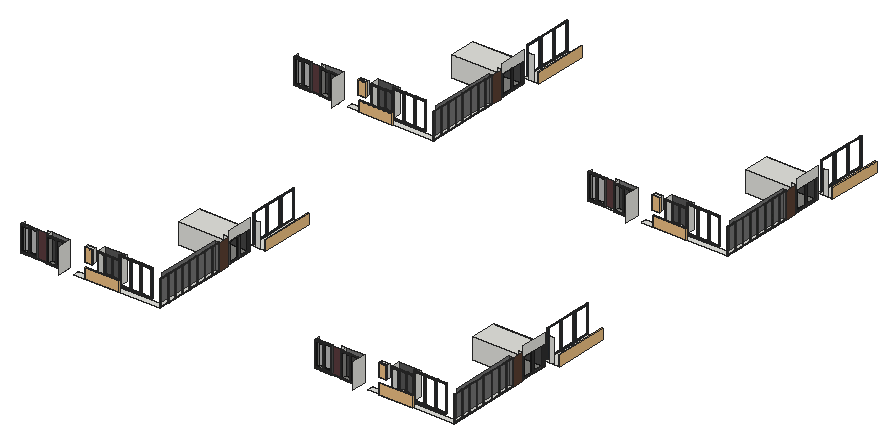
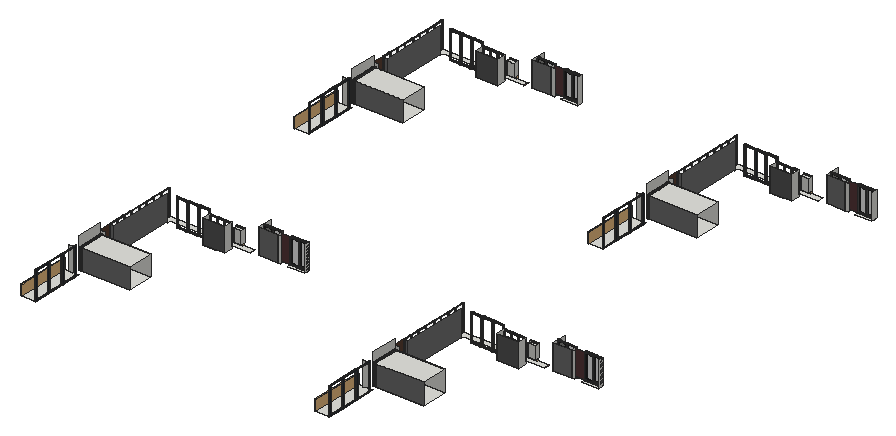
# SketchUp Ruby script. Lengths in inches.
U = 1.inch
M = Sketchup.active_model
def pt(a) = Geom::Point3d.new(a.map { |v| v * U })
def face(e, loops, mat)
  f = e.add_face(loops[0].map { |a| pt(a) })
  loops[1..].each { |l| e.add_face(l.map { |a| pt(a) }).erase! }
  f.material = f.back_material = mat if mat
  f
end
# faces: each face lists its corners as indices into pts; further lists are holes
def faces(e, pts, list, mat = nil) = list.each { |f| face(e, (f[0].is_a?(Array) ? f : [f]).map { |l| l.map { |i| pts[i] } }, mat) }
# xy, xz, yz: faces in a plane at the given z, y or x. An outline is a flat list of corners, or four numbers for a rectangle; further outlines are holes
def ring(l) = l.size == 4 ? [[l[0], l[1]], [l[2], l[1]], [l[2], l[3]], [l[0], l[3]]] : l.each_slice(2).to_a
def flat(e, list, mat, &to3) = list.each { |f| face(e, (f[0].is_a?(Array) ? f : [f]).map { |l| ring(l).map { |u, v| to3.(u, v) } }, mat) }
def xy(e, z, list, mat = nil) = flat(e, list, mat) { |x, y| [x, y, z] }
def xz(e, y, list, mat = nil) = flat(e, list, mat) { |x, z| [x, y, z] }
def yz(e, x, list, mat = nil) = flat(e, list, mat) { |y, z| [x, y, z] }
def lines(e, pts, list) = list.each { |a, b| e.add_line(pt(pts[a]), pt(pts[b])) }
# prism: a flat outline (further loops are holes) pulled along v
def prism(e, loops, v, mat = nil)
  f = face(e, loops, mat); d = Geom::Vector3d.new(v.map { |x| x * U })
  f.pushpull(f.normal.samedirection?(d) ? d.length : -d.length)
end
def box(e, o, s, mat = nil) = prism(e, [[o, [o[0] + s[0], o[1], o[2]], [o[0] + s[0], o[1] + s[1], o[2]], [o[0], o[1] + s[1], o[2]]]], [0, 0, s[2]], mat)
def at(x, y, z, deg = 0) = Geom::Transformation.translation(pt([x, y, z])) * Geom::Transformation.rotation(ORIGIN, Z_AXIS, deg.degrees)
def axes(o, x, y, z) = Geom::Transformation.new([*x, 0, *y, 0, *z, 0, *pt(o).to_a, 1])
def part(name) = M.definitions.add(name)
# library, detail: a bought-in or finely detailed component or shape, given as its bounding box
def library(name, o, s) = part(name).tap { |d| box(d.entities, o, s) }
def detail(e, o, s) = box(e.add_group.entities, o, s)
def put(e, d, t, mat = nil) = e.add_instance(d, t).tap { |i| i.material = mat if mat }
def group(e, t, mat = nil) = e.add_group.tap { |g| g.transformation = t; g.material = mat if mat }.entities
root = M.entities
M.materials.add("Glass_Tinted_Gray").color = [0, 0, 0]
M.materials["Glass_Tinted_Gray"].alpha = 0.125
M.materials.add("Glazing").color = [128, 128, 128]
M.materials["Glazing"].alpha = 0.05
M.materials.add("Powdercoating").color = [41, 44, 40]
M.materials.add("Wine2").color = [0, 0, 0]
M.materials["Wine2"].alpha = 0
M.materials.add("[0130_Gainsboro]").color = [39, 45, 50]
M.materials.add("[0135_DarkGray]").color = [81, 81, 81]
M.materials.add("[Color M05]").color = [114, 114, 114]
M.materials.add("[Color M06]").color = [86, 86, 86]
M.materials.add("[Granite Brown]").color = [89, 59, 61]
M.materials.add("[Granite Brown]1").color = [89, 63, 50]
M.materials.add("[Mirror 02]").color = [229, 229, 229]
M.materials.add("[Terrazzo Light Blue]").color = [196, 214, 227]
c1 = part("Framed glazing panel")
xy(c1.entities,0,[[0,-0.98,43.07,0],[0,0,43.07,1.4]],"[0130_Gainsboro]")
xy(c1.entities,0.3,[[0.3,-1.43,42.77,-0.98]],"[0130_Gainsboro]")
xy(c1.entities,2.95,[[2.95,-1.43,40.12,-0.63],[2.95,-0.63,40.12,0],[2.95,0,40.12,0.64],[2.95,0.64,40.12,1.4]],"[0130_Gainsboro]")
xy(c1.entities,3.54,[[3.54,-0.63,39.53,0],[3.54,0,39.53,0.64]],"[0130_Gainsboro]")
xy(c1.entities,111.8125,[[3.54,-0.63,39.53,0],[3.54,0,39.53,0.64]],"[0130_Gainsboro]")
xy(c1.entities,112.4,[[2.95,-1.43,40.12,-0.63],[2.95,-0.63,40.12,0],[2.95,0,40.12,0.64],[2.95,0.64,40.12,1.4]],"[0130_Gainsboro]")
xy(c1.entities,115.05,[[0.3,-1.43,42.77,-0.98]],"[0130_Gainsboro]")
xy(c1.entities,115.35,[[0,-0.98,43.07,0],[0,0,43.07,1.4]],"[0130_Gainsboro]")
xz(c1.entities,-1.43,[[[0.3,0.3,42.77,115.05],[2.95,2.95,40.12,112.4]]],"[0130_Gainsboro]")
xz(c1.entities,-0.98,[[[0,0,43.07,115.35],[0.3,0.3,42.77,115.05]]],"[0130_Gainsboro]")
xz(c1.entities,-0.63,[[[2.95,2.95,40.12,112.4],[3.54,3.54,39.53,111.8125]]],"[0130_Gainsboro]")
xz(c1.entities,0,[[3.54,3.54,39.53,111.8125]],"Wine2")
xz(c1.entities,0,[[[0,0,43.07,115.35],[2.95,2.95,40.12,112.4]],[[2.95,2.95,40.12,112.4],[3.54,3.54,39.53,111.8125]]],"[0130_Gainsboro]")
xz(c1.entities,0.64,[[[2.95,2.95,40.12,112.4],[3.54,3.54,39.53,111.8125]]],"[0130_Gainsboro]")
xz(c1.entities,1.4,[[[0,0,43.07,115.35],[2.95,2.95,40.12,112.4]]],"[0130_Gainsboro]")
yz(c1.entities,0,[[-0.98,0,0,115.35],[0,0,1.4,115.35]],"[0130_Gainsboro]")
yz(c1.entities,0.3,[[-1.43,0.3,-0.98,115.05]],"[0130_Gainsboro]")
yz(c1.entities,2.95,[[-1.43,2.95,-0.63,112.4],[-0.63,2.95,0,112.4],[0,2.95,0.64,112.4],[0.64,2.95,1.4,112.4]],"[0130_Gainsboro]")
yz(c1.entities,3.54,[[-0.63,3.54,0,111.8125],[0,3.54,0.64,111.8125]],"[0130_Gainsboro]")
yz(c1.entities,39.53,[[-0.63,3.54,0,111.8125],[0,3.54,0.64,111.8125]],"[0130_Gainsboro]")
yz(c1.entities,40.12,[[-1.43,2.95,-0.63,112.4],[-0.63,2.95,0,112.4],[0,2.95,0.64,112.4],[0.64,2.95,1.4,112.4]],"[0130_Gainsboro]")
yz(c1.entities,42.77,[[-1.43,0.3,-0.98,115.05]],"[0130_Gainsboro]")
yz(c1.entities,43.07,[[-0.98,0,0,115.35],[0,0,1.4,115.35]],"[0130_Gainsboro]")
c2 = part("Glazed panel assembly")
put(c2.entities,c1,axes([90.57,1.43,0],[1.05148,0,0],[0,1,0],[0,0,1]))
put(c2.entities,c1,axes([0,1.43,0],[1.05148,0,0],[0,1,0],[0,0,1]))
put(c2.entities,c1,axes([45.29,1.43,0],[1.05148,0,0],[0,1,0],[0,0,1]))
c3 = part("Group\#15")
xy(c3.entities,0,[[0,-55.94,0.71,45.94]])
xy(c3.entities,0.2,[[0,-55.94,0.47,45.94],[0.47,45.94,0.71,46.42]])
xy(c3.entities,2.36,[[0.47,-55.94,0.71,46.42]])
xz(c3.entities,-55.94,[[0,0,0.71,0,0.71,2.36,0.47,2.36,0.47,0.2,0,0.2]])
xz(c3.entities,45.94,[[0,0,0.71,0.2]])
xz(c3.entities,46.42,[[0.47,0.2,0.71,2.36]])
yz(c3.entities,0,[[-55.94,0,45.94,0.2]])
yz(c3.entities,0.47,[[-55.94,0.2,46.42,2.36]])
yz(c3.entities,0.71,[[-55.94,0,45.94,0,45.94,0.2,46.42,0.2,46.42,2.36,-55.94,2.36]])
c4 = part("Group\#7")
xy(c4.entities,0,[[0,-59.09,0.71,45.94]])
xy(c4.entities,0.2,[[0,-59.09,0.47,45.94],[0.47,45.94,0.71,46.42]])
xy(c4.entities,2.36,[[0.47,-59.09,0.71,46.42]])
xz(c4.entities,-59.09,[[0,0,0.71,0,0.71,2.36,0.47,2.36,0.47,0.2,0,0.2]])
xz(c4.entities,45.94,[[0,0,0.71,0.2]])
xz(c4.entities,46.42,[[0.47,0.2,0.71,2.36]])
yz(c4.entities,0,[[-59.09,0,45.94,0.2]])
yz(c4.entities,0.47,[[-59.09,0.2,46.42,2.36]])
yz(c4.entities,0.71,[[-59.09,0,45.94,0,45.94,0.2,46.42,0.2,46.42,2.36,-59.09,2.36]])
c5 = part("Group\#16")
prism(c5.entities,[[[0.47,-56.18,0.2],[0,-56.18,0.2],[0,-56.18,0],[0.71,-56.18,0],[0.71,-56.18,2.36],[0.47,-56.18,2.36]]],[0,28.68,0])
c6 = part("Group\#10")
box(c6.entities,[-0.73,0,0],[27.99,0.55,102.05])
c7 = part("Group\#18")
xy(c7.entities,0,[[0.47,-56.18,0.47,-55.47,0,-55.47,0,-28.21,1.18,-28.21,1.18,-56.18]])
xy(c7.entities,0.2,[[0.71,-56.18,1.18,-28.21],[0,-55.47,0.47,-28.21],[0.47,-28.21,0.71,-27.74]])
xy(c7.entities,2.36,[[0.47,-56.18,0.71,-27.74]])
xz(c7.entities,-56.18,[[0.47,0,1.18,0,1.18,0.2,0.71,0.2,0.71,2.36,0.47,2.36]])
xz(c7.entities,-55.47,[[0,0,0.47,0.2]])
xz(c7.entities,-28.21,[[0,0,1.18,0.2]])
xz(c7.entities,-27.74,[[0.47,0.2,0.71,2.36]])
yz(c7.entities,0,[[-55.47,0,-28.21,0.2]])
yz(c7.entities,0.47,[[-56.18,0,-55.47,0.2],[-56.18,0.2,-27.74,2.36]])
yz(c7.entities,0.71,[[-56.18,0.2,-27.74,2.36]])
yz(c7.entities,1.18,[[-56.18,0,-28.21,0.2]])
c8 = part("Group\#34")
xy(c8.entities,0,[[-20.45,0,7.76,1.22]])
xy(c8.entities,0.06,[[-20.39,0.06,7.7,1.22]])
xy(c8.entities,0.47,[[-19.98,0,7.28,0.06]])
xy(c8.entities,101.89,[[-19.98,0,7.28,0.06]])
xy(c8.entities,102.3,[[-20.39,0.06,7.7,1.22]])
xy(c8.entities,102.36,[[-20.45,0,7.76,1.22]])
xz(c8.entities,0,[[[-20.45,0,7.76,102.36],[-19.98,0.47,7.28,101.89]]])
xz(c8.entities,0.06,[[[-20.39,0.06,7.7,102.3],[-19.98,0.47,7.28,101.89]]])
xz(c8.entities,1.22,[[[-20.45,0,7.76,102.36],[-20.39,0.06,7.7,102.3]]])
yz(c8.entities,-20.45,[[0,0,1.22,102.36]])
yz(c8.entities,-20.39,[[0.06,0.06,1.22,102.3]])
yz(c8.entities,-19.98,[[0,0.47,0.06,101.89]])
yz(c8.entities,7.28,[[0,0.47,0.06,101.89]])
yz(c8.entities,7.7,[[0.06,0.06,1.22,102.3]])
yz(c8.entities,7.76,[[0,0,1.22,102.36]])
c9 = part("Group\#6")
put(c9.entities,c3,axes([27.97,0,7.875],[1,0,0],[0,0,-1],[0,1,0]),"Powdercoating")
put(c9.entities,c4,axes([0.71,0,6.8],[-1,0,0],[0,0,-0.97687],[0,1,0]),"Powdercoating")
put(c9.entities,c5,axes([-27.5,0,-38.07],[0,0,-1],[-1,0,0],[0,1,0]),"Powdercoating")
put(c9.entities,c6,at(1.12,0.35,-38.39),"Glazing")
put(c9.entities,c7,axes([-27.5,0,63.35],[0,0,1],[-1,0,0],[0,1,0]),"Powdercoating")
put(c9.entities,c8,at(20.6875,1.0625,-38.54),"Powdercoating")
c10 = part("Sliding door assembly")
put(c10.entities,c9,at(-1.18,4.5,38.86))
g1 = group(c10.entities,at(84.74,4.5,38.86))
put(g1,c3,axes([-27.97,0,7.875],[-1,0,0],[0,0,-1],[0,1,0]),"Powdercoating")
put(g1,c4,axes([-0.71,0,6.8],[1,0,0],[0,0,-0.97687],[0,1,0]),"Powdercoating")
put(g1,c5,axes([27.5,0,-38.07],[0,0,-1],[1,0,0],[0,1,0]),"Powdercoating")
put(g1,c6,axes([-1.12,0.35,-38.39],[-1,0,0],[0,1,0],[0,0,1]),"Glazing")
put(g1,c7,axes([27.5,0,63.35],[0,0,1],[1,0,0],[0,1,0]),"Powdercoating")
put(g1,c8,axes([-20.6875,1.0625,-38.54],[-1,0,0],[0,1,0],[0,0,1]),"Powdercoating")
g2 = group(c10.entities,at(56.0625,4.5,38.86))
put(g2,c3,axes([-27.97,0,7.875],[-1,0,0],[0,0,-1],[0,1,0]),"Powdercoating")
put(g2,c5,axes([27.5,0,-38.07],[0,0,-1],[1,0,0],[0,1,0]),"Powdercoating")
put(g2,c6,axes([-1.12,0.35,-38.39],[-1,0,0],[0,1,0],[0,0,1]),"Glazing")
put(g2,c7,axes([27.5,0,63.35],[0,0,1],[1,0,0],[0,1,0]),"Powdercoating")
put(g2,c8,axes([-20.6875,1.0625,-38.54],[-1,0,0],[0,1,0],[0,0,1]),"Powdercoating")
g3 = group(g2,at(-0.71,0,6.8),"Powdercoating")
xy(g3,-45.34,[[0.47,0.2,0.71,2.36]])
xy(g3,-44.88,[[0,0,0.71,0.2]])
xy(g3,57.73,[[0,0,0.71,0,0.71,2.36,0.47,2.36,0.47,0.2,0,0.2]])
xz(g3,0,[[0,-44.88,0.71,57.73]])
xz(g3,0.2,[[0.47,-45.34,0.71,-44.88],[0,-44.88,0.47,57.73]])
xz(g3,2.36,[[0.47,-45.34,0.71,57.73]])
yz(g3,0,[[0,-44.88,0.2,57.73]])
yz(g3,0.47,[[0.2,-45.34,2.36,57.73]])
yz(g3,0.71,[[0.2,-45.34,2.36,-45.34,2.36,57.73,0,57.73,0,-44.88,0.2,-44.88]])
put(c10.entities,c9,axes([-33.94,4.5,38.86],[1.14218,0,0],[0,1,0],[0,0,1]))
c11 = part("sliding door")
put(c11.entities,c10,at(0,-4.5,-0.08))
c12 = library("Glass Railing",[0,0,0],[139.5,4.76,42])
c13 = part("PENTEK_RP Fineline 50S_Sliding_DoorCase_E1")
box(c13.entities,[0,0,0],[1.51,3.66,99.27],"[0135_DarkGray]")
c14 = part("PENTEK_RP Fineline 50S_SlidingDooe_Case_E2")
box(c14.entities,[0,0,0],[96.25,3.66,1.51],"[0135_DarkGray]")
c15 = part("pentek_RP Fineline 50S_SlidingDoor_Case")
put(c15.entities,c13,at(97.76,0,0))
put(c15.entities,c14,at(1.51,0,0))
put(c15.entities,c13,at(0,0,0))
put(c15.entities,c14,at(1.51,0,97.76))
c16 = part("PENTEK_RP Fineline 50S_SlidingDoor_GlazingBead_2")
box(c16.entities,[0,0,0],[0.56,0.59,94.39],"[0135_DarkGray]")
c17 = part("PENTEK_RP Fineline 50S_SlidingDoor_Glass")
box(c17.entities,[0,0,0],[46.58,0.16,94.39],"Glass_Tinted_Gray")
c18 = part("PENTEK_RP Fineline 50S_SlidingDoor_GlazingBead")
box(c18.entities,[0,0,0],[45.47,0.59,0.56],"[0135_DarkGray]")
c19 = part("PENTEK_RP Fineline 50S_SlidingDoor_Leaf_E1")
xy(c19.entities,0,[[0,0,0.93,1.97],[0.93,1.57,1.49,1.97]],"[0135_DarkGray]")
xy(c19.entities,96.25,[[0,0,0.93,0,0.93,1.57,1.49,1.57,1.49,1.97,0,1.97]],"[0135_DarkGray]")
xz(c19.entities,0,[[0,0,0.93,96.25]],"[0135_DarkGray]")
xz(c19.entities,1.57,[[0.93,0,1.49,95.32],[0.93,95.32,1.49,96.25]],"[0135_DarkGray]")
xz(c19.entities,1.97,[[0,0,1.49,96.25]],"[0135_DarkGray]")
yz(c19.entities,0,[[0,0,1.97,96.25]],"[0135_DarkGray]")
yz(c19.entities,0.93,[[0,0,1.57,0.93],[0,0.93,1.57,95.32],[0,95.32,1.57,96.25]],"[0135_DarkGray]")
yz(c19.entities,1.49,[[1.57,0,1.97,95.32],[1.57,95.32,1.97,96.25]],"[0135_DarkGray]")
c20 = part("PENTEK_RP Fineline 50S_SlidingDoor_Leaf_E2")
xy(c20.entities,0,[[0,0,0,1.57,0.56,1.57,0.56,1.97,46.02,1.97,46.02,1.57,46.58,1.57,46.58,0]],"[0135_DarkGray]")
xy(c20.entities,0.93,[[0,0,46.58,1.57]],"[0135_DarkGray]")
xy(c20.entities,1.49,[[0.56,1.57,46.02,1.97]],"[0135_DarkGray]")
xz(c20.entities,0,[[0,0,46.58,0.93]],"[0135_DarkGray]")
xz(c20.entities,1.57,[[0,0,0.56,0.93],[46.02,0,46.58,0.93],[0.56,0.93,46.02,1.49]],"[0135_DarkGray]")
xz(c20.entities,1.97,[[0.56,0,46.02,1.49]],"[0135_DarkGray]")
yz(c20.entities,0,[[0,0,1.57,0.93]],"[0135_DarkGray]")
yz(c20.entities,0.56,[[1.57,0,1.97,0.93],[1.57,0.93,1.97,1.49]],"[0135_DarkGray]")
yz(c20.entities,46.02,[[1.57,0,1.97,0.93],[1.57,0.93,1.97,1.49]],"[0135_DarkGray]")
yz(c20.entities,46.58,[[0,0,1.57,0.93]],"[0135_DarkGray]")
c21 = part("PENTEK_RP Fineline S_SlidingDoor_Leaf1")
put(c21.entities,c16,at(0.93,0,0.93))
put(c21.entities,c16,at(46.96,0,0.93))
put(c21.entities,c17,at(1.49,1.42,0.93))
put(c21.entities,c18,at(1.49,0,0.93))
put(c21.entities,c17,at(1.49,0.59,0.93),"[Terrazzo Light Blue]")
put(c21.entities,c19,at(0,0,0))
put(c21.entities,c19,axes([48.44,0,0],[-1,0,0],[0,1,0],[0,0,1]))
put(c21.entities,c20,axes([0.93,0,96.25],[1,0,0],[0,1,0],[0,0,-1]))
put(c21.entities,c20,at(0.93,0,0))
put(c21.entities,c18,at(1.49,0,94.77))
c22 = part("PENTEK_RP Fineline 50S_SlidingDoor_Leaf2")
put(c22.entities,c17,at(1.49,1.42,0.93))
put(c22.entities,c18,at(1.49,0,94.77))
put(c22.entities,c16,at(46.96,0,0.93))
put(c22.entities,c17,at(1.49,0.59,0.93),"[Mirror 02]")
put(c22.entities,c16,at(0.93,0,0.93))
put(c22.entities,c19,at(0,0,0))
put(c22.entities,c19,axes([48.44,0,0],[-1,0,0],[0,1,0],[0,0,1]))
put(c22.entities,c18,at(1.49,0,0.93))
put(c22.entities,c20,axes([0.93,0,96.25],[1,0,0],[0,1,0],[0,0,-1]))
put(c22.entities,c20,at(0.93,0,0))
c23 = part("PENTEK - Slimmest Steel Sliding Door / Window\#1")
put(c23.entities,c15,at(0,-1.88,-0.09))
put(c23.entities,c21,at(1.51,-2.27,1.42))
put(c23.entities,c22,at(49.32,-0.3,1.42))
c24 = library("Klein+raam",[128.36,12.7,0],[19.68,5.51,55.12])
xy(root,1023.2,[[646.53,1835.1875,662.84,1873.375],[662.84,1835.1875,664.52,1873.375],[664.52,1835.1875,715.63,1873.375],[1864.72,1835.1875,1881.02,1873.375],[1881.02,1835.1875,1882.71,1873.375],
  [1882.71,1835.1875,1933.82,1873.375],[646.53,3249.875,662.84,3288.0625],[662.84,3249.875,664.52,3288.0625],[664.52,3249.875,715.63,3288.0625],[1864.72,3249.875,1881.02,3288.0625],
  [1881.02,3249.875,1882.71,3288.0625],[1882.71,3249.875,1933.82,3288.0625]])
xy(root,1023.51,[[625.7,1835.1875,646.53,1873.375],[1843.88,1835.1875,1864.72,1873.375],[625.7,3249.875,646.53,3288.0625],[1843.88,3249.875,1864.72,3288.0625]])
xy(root,1026.6875,[[557.88,1799.9375,913.875,1799.9375,913.875,2108.8,894.3125,2108.8,894.3125,1835.1875,890.875,1835.1875,890.875,1822.9375,557.88,1822.9375],[1776.07,1799.9375,2132.0625,1799.9375,2132.0625,2108.8,2112.5,2108.8,2112.5,1835.1875,2109.0625,1835.1875,2109.0625,1822.9375,1776.07,1822.9375],[661.4375,1822.9375,704.25,1833.75],[1879.625,1822.9375,1922.4375,1833.75],[557.88,3214.625,913.875,3214.625,913.875,3523.49,894.3125,3523.49,894.3125,3249.875,890.875,3249.875,890.875,3237.625,557.88,3237.625],
  [1776.07,3214.625,2132.0625,3214.625,2132.0625,3523.49,2112.5,3523.49,2112.5,3249.875,2109.0625,3249.875,2109.0625,3237.625,1776.07,3237.625],[661.4375,3237.625,704.25,3248.4375],[1879.625,3237.625,1922.4375,3248.4375]])
xy(root,1026.6875,[[557.4,1799.9375,557.88,1822.9375],[1775.59,1799.9375,1776.07,1822.9375],[557.4,3214.625,557.88,3237.625],[1775.59,3214.625,1776.07,3237.625]],"[Granite Brown]")
xy(root,1029.4375,[[334.58,1799.9375,403.69,1822.9375],[403.69,1799.9375,431.33,1806.5625],[431.33,1799.9375,523.04,1799.9375,523.04,1822.9375,446.15,1822.9375,446.15,1806.5625,431.33,1806.5625],[1552.77,1799.9375,1621.88,1822.9375],[1621.88,1799.9375,1649.52,1806.5625],
  [1649.52,1799.9375,1741.23,1799.9375,1741.23,1822.9375,1664.33,1822.9375,1664.33,1806.5625,1649.52,1806.5625],[431.33,1806.5625,446.15,1822.9375],[1649.52,1806.5625,1664.33,1822.9375],[334.58,3214.625,403.69,3237.625],[403.69,3214.625,431.33,3221.25],
  [431.33,3214.625,523.04,3214.625,523.04,3237.625,446.15,3237.625,446.15,3221.25,431.33,3221.25],[1552.77,3214.625,1621.88,3237.625],[1621.88,3214.625,1649.52,3221.25],[1649.52,3214.625,1741.23,3214.625,1741.23,3237.625,1664.33,3237.625,1664.33,3221.25,1649.52,3221.25],[431.33,3221.25,446.15,3237.625],
  [1649.52,3221.25,1664.33,3237.625]])
xy(root,1031.36,[[704.25,2156.01,913.875,2266.33],[1922.4375,2156.01,2132.0625,2266.33],[704.25,3570.7,913.875,3681.01],[1922.4375,3570.7,2132.0625,3681.01]])
xy(root,1034.8125,[[890.875,2295.875,954.6875,2518.89],[2109.0625,2295.875,2172.875,2518.89],[890.875,3710.5625,954.6875,3933.57],[2109.0625,3710.5625,2172.875,3933.57]])
xy(root,1064.45,[[571.45,1835.1875,603.76,1854.3125],[1789.64,1835.1875,1821.95,1854.3125],[571.45,3249.875,603.76,3269],[1789.64,3249.875,1821.95,3269]])
xy(root,1116.73,[[571.45,1835.1875,603.76,1854.3125],[1789.64,1835.1875,1821.95,1854.3125],[571.45,3249.875,603.76,3269],[1789.64,3249.875,1821.95,3269]])
xy(root,1117.04,[[704.25,2156.01,913.875,2266.33],[1922.4375,2156.01,2132.0625,2266.33],[704.25,3570.7,913.875,3681.01],[1922.4375,3570.7,2132.0625,3681.01]])
xz(root,1806.5625,[[403.77,1029.4375,446.15,1029.4375,446.15,1134,404.29,1134],[1621.96,1029.4375,1664.33,1029.4375,1664.33,1134,1622.48,1134]],"[Granite Brown]")
xz(root,1822.9375,[[431.33,1029.4375,446.15,1134],[1649.52,1029.4375,1664.33,1134]])
xz(root,1822.9375,[[446.15,1029.4375,523.04,1134],[1664.33,1029.4375,1741.23,1134]],"[Color M05]")
xz(root,1854.3125,[[571.45,1064.45,603.76,1116.73],[1789.64,1064.45,1821.95,1116.73]])
xz(root,1873.375,[[646.53,1023.2,715.63,1023.2,715.63,1121.33,625.7,1121.33,625.7,1023.51,646.53,1023.51],[1864.72,1023.2,1933.82,1023.2,1933.82,1121.33,1843.88,1121.33,1843.88,1023.51,1864.72,1023.51]],"[Color M06]")
xz(root,2108.8,[[894.3125,1026.6875,913.875,1134],[2112.5,1026.6875,2132.0625,1134]],"[Color M05]")
xz(root,2156.01,[[704.25,1031.36,894.3125,1117.04],[894.3125,1031.36,913.875,1117.04],[1922.4375,1031.36,2112.5,1117.04],[2112.5,1031.36,2132.0625,1117.04],[894.3125,1117.04,913.875,1134],
  [2112.5,1117.04,2132.0625,1134]])
xz(root,2266.33,[[704.25,1031.36,913.875,1117.04],[1922.4375,1031.36,2132.0625,1117.04]],"[Color M05]")
xz(root,2295.875,[[913.875,1034.8125,930.75,1134],[2132.0625,1034.8125,2148.9375,1134]])
xz(root,3221.25,[[403.77,1029.4375,446.15,1029.4375,446.15,1134,404.29,1134],[1621.96,1029.4375,1664.33,1029.4375,1664.33,1134,1622.48,1134]],"[Granite Brown]")
xz(root,3237.625,[[431.33,1029.4375,446.15,1134],[1649.52,1029.4375,1664.33,1134]])
xz(root,3237.625,[[446.15,1029.4375,523.04,1134],[1664.33,1029.4375,1741.23,1134]],"[Color M05]")
xz(root,3269,[[571.45,1064.45,603.76,1116.73],[1789.64,1064.45,1821.95,1116.73]])
xz(root,3288.0625,[[646.53,1023.2,715.63,1023.2,715.63,1121.33,625.7,1121.33,625.7,1023.51,646.53,1023.51],[1864.72,1023.2,1933.82,1023.2,1933.82,1121.33,1843.88,1121.33,1843.88,1023.51,1864.72,1023.51]],"[Color M06]")
xz(root,3523.49,[[894.3125,1026.6875,913.875,1134],[2112.5,1026.6875,2132.0625,1134]],"[Color M05]")
xz(root,3570.7,[[704.25,1031.36,894.3125,1117.04],[894.3125,1031.36,913.875,1117.04],[1922.4375,1031.36,2112.5,1117.04],[2112.5,1031.36,2132.0625,1117.04],[894.3125,1117.04,913.875,1134],
  [2112.5,1117.04,2132.0625,1134]])
xz(root,3681.01,[[704.25,1031.36,913.875,1117.04],[1922.4375,1031.36,2132.0625,1117.04]],"[Color M05]")
xz(root,3710.5625,[[913.875,1034.8125,930.75,1134],[2132.0625,1034.8125,2148.9375,1134]])
yz(root,334.58,[[1799.9375,1029.4375,1822.9375,1134],[3214.625,1029.4375,3237.625,1134]])
yz(root,446.15,[[1806.5625,1029.4375,1822.9375,1134],[3221.25,1029.4375,3237.625,1134]])
yz(root,523.04,[[1763.25,1029.4375,1822.9375,1134],[3177.9375,1029.4375,3237.625,1134]])
yz(root,571.45,[[1835.1875,1064.45,1854.3125,1116.73],[3249.875,1064.45,3269,1116.73]])
yz(root,603.76,[[1835.1875,1064.45,1854.3125,1116.73],[3249.875,1064.45,3269,1116.73]])
yz(root,625.7,[[1835.1875,1023.51,1873.375,1121.33],[3249.875,1023.51,3288.0625,1121.33]])
yz(root,646.53,[[1835.1875,1023.2,1873.375,1023.51],[3249.875,1023.2,3288.0625,1023.51]])
yz(root,715.63,[[1835.1875,1023.2,1873.375,1121.33],[3249.875,1023.2,3288.0625,1121.33]])
yz(root,894.3125,[[1835.1875,1026.6875,2108.8,1134],[3249.875,1026.6875,3523.49,1134]],"[Color M05]")
yz(root,913.875,[[2156.01,1117.04,2266.33,1157.36],[3570.7,1117.04,3681.01,1157.36]])
yz(root,913.875,[[2108.8,1026.6875,2148.83,1134],[3523.49,1026.6875,3563.51,1134]],"[Granite Brown]1")
yz(root,1552.77,[[1799.9375,1029.4375,1822.9375,1134],[3214.625,1029.4375,3237.625,1134]])
yz(root,1664.33,[[1806.5625,1029.4375,1822.9375,1134],[3221.25,1029.4375,3237.625,1134]])
yz(root,1741.23,[[1763.25,1029.4375,1822.9375,1134],[3177.9375,1029.4375,3237.625,1134]])
yz(root,1789.64,[[1835.1875,1064.45,1854.3125,1116.73],[3249.875,1064.45,3269,1116.73]])
yz(root,1821.95,[[1835.1875,1064.45,1854.3125,1116.73],[3249.875,1064.45,3269,1116.73]])
yz(root,1843.88,[[1835.1875,1023.51,1873.375,1121.33],[3249.875,1023.51,3288.0625,1121.33]])
yz(root,1864.72,[[1835.1875,1023.2,1873.375,1023.51],[3249.875,1023.2,3288.0625,1023.51]])
yz(root,1933.82,[[1835.1875,1023.2,1873.375,1121.33],[3249.875,1023.2,3288.0625,1121.33]])
yz(root,2112.5,[[1835.1875,1026.6875,2108.8,1134],[3249.875,1026.6875,3523.49,1134]],"[Color M05]")
yz(root,2132.0625,[[2156.01,1117.04,2266.33,1157.36],[3570.7,1117.04,3681.01,1157.36]])
yz(root,2132.0625,[[2108.8,1026.6875,2148.83,1134],[3523.49,1026.6875,3563.51,1134]],"[Granite Brown]1")
p = [[1955.15,1799.9375,1024.15],[1955.15,1799.36,1024.15],[1955.15,1799.36,1026.6875],[736.96,1799.9375,1024.15],[736.96,1799.36,1024.15],[736.96,1799.36,1026.6875],
  [1955.15,3214.05,1026.6875],[1955.15,3214.05,1024.15],[1955.15,3214.625,1024.15],[736.96,3214.05,1026.6875],[736.96,3214.05,1024.15],[736.96,3214.625,1024.15]]
lines(root,p,[[0,1],[2,1],[3,4],[5,4],[6,7],[8,7],[9,10],[11,10]])
put(root,c2,at(1933.82,1835.1875,1023.2))
put(root,c2,at(715.63,1835.1875,1023.2))
put(root,c2,at(1933.82,3249.875,1023.2))
put(root,c2,at(715.63,3249.875,1023.2))
put(root,c11,axes([2132.0625,1844.13,1026.6875],[0,1.302,0],[-1,0,0],[0,0,1.03877]))
put(root,c12,at(1822.95,1797.87,1026.6875))
put(root,c11,axes([913.875,1844.13,1026.6875],[0,1.302,0],[-1,0,0],[0,0,1.03877]))
put(root,c12,at(604.76,1797.87,1026.6875))
put(root,c11,axes([2132.0625,3258.81,1026.6875],[0,1.302,0],[-1,0,0],[0,0,1.03877]))
put(root,c12,at(1822.95,3212.55,1026.6875))
put(root,c11,axes([913.875,3258.81,1026.6875],[0,1.302,0],[-1,0,0],[0,0,1.03877]))
put(root,c12,at(604.76,3212.55,1026.6875))
put(root,c11,axes([2131,1997.73,1027.42],[0,1.302,0],[-1,0,0],[0,0,1.03877]))
put(root,c11,axes([912.8125,1997.73,1027.42],[0,1.302,0],[-1,0,0],[0,0,1.03877]))
put(root,c11,axes([2131,3412.42,1027.42],[0,1.302,0],[-1,0,0],[0,0,1.03877]))
put(root,c11,axes([912.8125,3412.42,1027.42],[0,1.302,0],[-1,0,0],[0,0,1.03877]))
put(root,c23,axes([1552.77,1805.65,1029.53],[0.69696,0,0],[0,2.51374,0],[0,0,1.054]))
put(root,c23,axes([334.58,1805.65,1029.53],[0.69696,0,0],[0,2.51374,0],[0,0,1.054]))
put(root,c23,axes([1552.77,3220.33,1029.53],[0.69696,0,0],[0,2.51374,0],[0,0,1.054]))
put(root,c23,axes([334.58,3220.33,1029.53],[0.69696,0,0],[0,2.51374,0],[0,0,1.054]))
put(root,c23,axes([1664.08,1798.37,1029.53],[0.77709,0,0],[0,0.88,0],[0,0,1.054]))
put(root,c23,axes([445.89,1798.37,1029.53],[0.77709,0,0],[0,0.88,0],[0,0,1.054]))
put(root,c23,axes([1664.08,3213.05,1029.53],[0.77709,0,0],[0,0.88,0],[0,0,1.054]))
put(root,c23,axes([445.89,3213.05,1029.53],[0.77709,0,0],[0,0.88,0],[0,0,1.054]))
put(root,c23,axes([2126.35,2154.96,1031.4375],[0,1.12181,0],[-2.51374,0,0],[0,0,0.87918]))
put(root,c23,axes([908.17,2154.96,1031.4375],[0,1.12181,0],[-2.51374,0,0],[0,0,0.87918]))
put(root,c23,axes([2126.35,3569.65,1031.4375],[0,1.12181,0],[-2.51374,0,0],[0,0,0.87918]))
put(root,c23,axes([908.17,3569.65,1031.4375],[0,1.12181,0],[-2.51374,0,0],[0,0,0.87918]))
put(root,c2,axes([2111.89,2309.55,1034.8125],[0,1.54079,0],[-1,0,0],[0,0,1]))
put(root,c12,axes([2172.875,2295.6875,1034.8125],[0,1.6,0],[-1,0,0],[0,0,1]))
put(root,c12,axes([954.6875,2295.6875,1034.8125],[0,1.6,0],[-1,0,0],[0,0,1]))
put(root,c2,axes([893.71,2309.55,1034.8125],[0,1.54079,0],[-1,0,0],[0,0,1]))
put(root,c12,axes([2172.875,3710.375,1034.8125],[0,1.6,0],[-1,0,0],[0,0,1]))
put(root,c2,axes([2111.89,3724.24,1034.8125],[0,1.54079,0],[-1,0,0],[0,0,1]))
put(root,c12,axes([954.6875,3710.375,1034.8125],[0,1.6,0],[-1,0,0],[0,0,1]))
put(root,c2,axes([893.71,3724.24,1034.8125],[0,1.54079,0],[-1,0,0],[0,0,1]))
put(root,c2,axes([1843.49,1835.1875,1034.83],[0.6649,0,0],[0,0.61,0],[0,0,0.74986]),"[Color M06]")
put(root,c2,axes([625.3,1835.1875,1034.83],[0.6649,0,0],[0,0.61,0],[0,0,0.74986]),"[Color M06]")
put(root,c2,axes([1843.49,3249.875,1034.83],[0.6649,0,0],[0,0.61,0],[0,0,0.74986]),"[Color M06]")
put(root,c2,axes([625.3,3249.875,1034.83],[0.6649,0,0],[0,0.61,0],[0,0,0.74986]),"[Color M06]")
put(root,c24,axes([1588.14,1826.55,1063.66],[1.58777,0,0],[0,0.68,0],[0,0,0.99202]))
put(root,c24,axes([369.95,1826.55,1063.66],[1.58777,0,0],[0,0.68,0],[0,0,0.99202]))
put(root,c24,axes([1588.14,3241.24,1063.66],[1.58777,0,0],[0,0.68,0],[0,0,0.99202]))
put(root,c24,axes([369.95,3241.24,1063.66],[1.58777,0,0],[0,0.68,0],[0,0,0.99202]))
